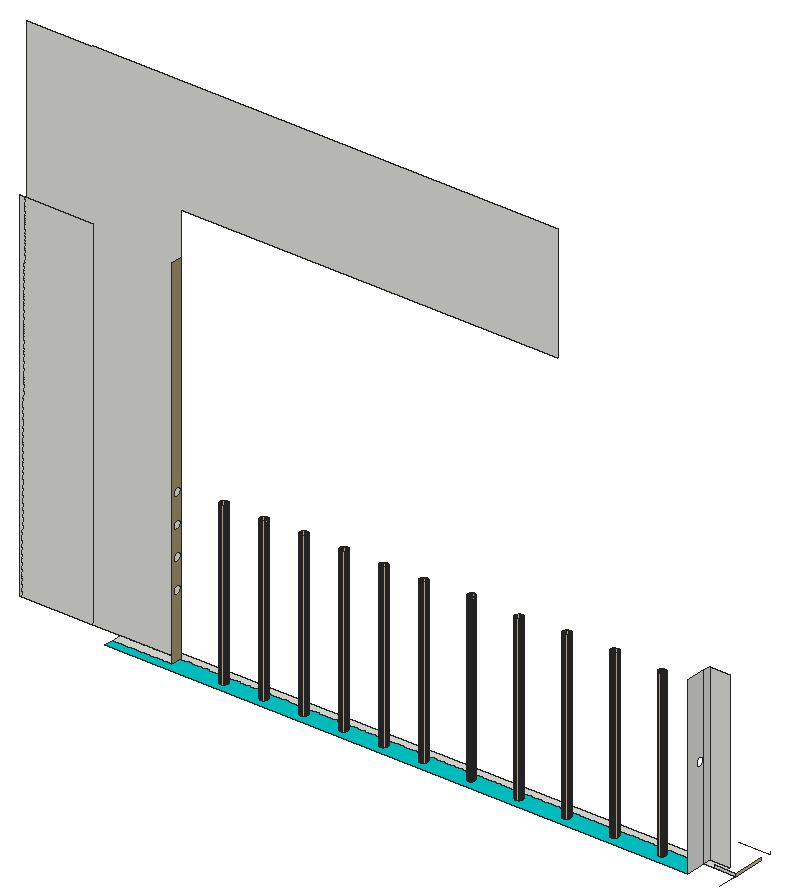
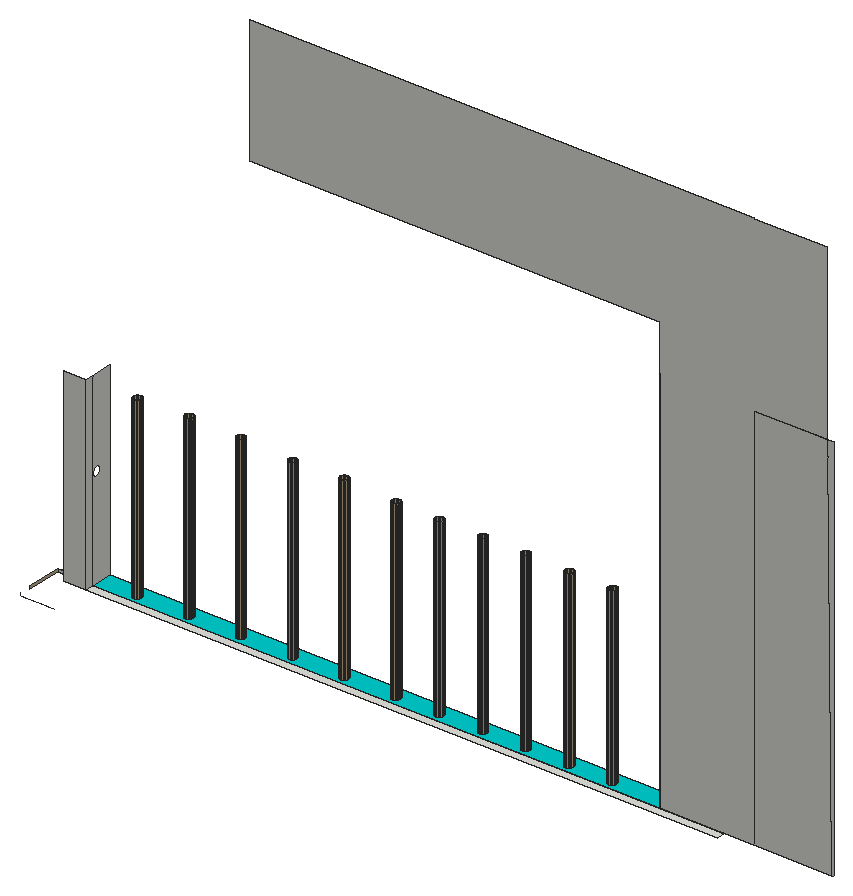
# SketchUp Ruby script. Lengths in inches.
U = 1.inch
M = Sketchup.active_model
def pt(a) = Geom::Point3d.new(a.map { |v| v * U })
def face(e, loops, mat)
  f = e.add_face(loops[0].map { |a| pt(a) })
  loops[1..].each { |l| e.add_face(l.map { |a| pt(a) }).erase! }
  f.material = f.back_material = mat if mat
  f
end
# faces: each face lists its corners as indices into pts; further lists are holes
def faces(e, pts, list, mat = nil) = list.each { |f| face(e, (f[0].is_a?(Array) ? f : [f]).map { |l| l.map { |i| pts[i] } }, mat) }
# xy, xz, yz: faces in a plane at the given z, y or x. An outline is a flat list of corners, or four numbers for a rectangle; further outlines are holes
def ring(l) = l.size == 4 ? [[l[0], l[1]], [l[2], l[1]], [l[2], l[3]], [l[0], l[3]]] : l.each_slice(2).to_a
def flat(e, list, mat, &to3) = list.each { |f| face(e, (f[0].is_a?(Array) ? f : [f]).map { |l| ring(l).map { |u, v| to3.(u, v) } }, mat) }
def xy(e, z, list, mat = nil) = flat(e, list, mat) { |x, y| [x, y, z] }
def xz(e, y, list, mat = nil) = flat(e, list, mat) { |x, z| [x, y, z] }
def yz(e, x, list, mat = nil) = flat(e, list, mat) { |y, z| [x, y, z] }
def lines(e, pts, list) = list.each { |a, b| e.add_line(pt(pts[a]), pt(pts[b])) }
# prism: a flat outline (further loops are holes) pulled along v
def prism(e, loops, v, mat = nil)
  f = face(e, loops, mat); d = Geom::Vector3d.new(v.map { |x| x * U })
  f.pushpull(f.normal.samedirection?(d) ? d.length : -d.length)
end
def box(e, o, s, mat = nil) = prism(e, [[o, [o[0] + s[0], o[1], o[2]], [o[0] + s[0], o[1] + s[1], o[2]], [o[0], o[1] + s[1], o[2]]]], [0, 0, s[2]], mat)
def at(x, y, z, deg = 0) = Geom::Transformation.translation(pt([x, y, z])) * Geom::Transformation.rotation(ORIGIN, Z_AXIS, deg.degrees)
def axes(o, x, y, z) = Geom::Transformation.new([*x, 0, *y, 0, *z, 0, *pt(o).to_a, 1])
def part(name) = M.definitions.add(name)
# library, detail: a bought-in or finely detailed component or shape, given as its bounding box
def library(name, o, s) = part(name).tap { |d| box(d.entities, o, s) }
def detail(e, o, s) = box(e.add_group.entities, o, s)
def put(e, d, t, mat = nil) = e.add_instance(d, t).tap { |i| i.material = mat if mat }
def group(e, t, mat = nil) = e.add_group.tap { |g| g.transformation = t; g.material = mat if mat }.entities
root = M.entities
M.materials.add("[Color H06]").color = [0, 204, 204]
M.materials.add("[Formica Beige]").color = [211, 187, 149]
M.materials.add("[Quartz Light Brown]").color = [199, 184, 152]
M.materials.add("[Wood Lumber ButtJoined]").color = [164, 152, 112]
xy(root,139.375,[[302.87,81.02,302.59,81.06,302.34,81.16,302.12,81.33,301.95,81.55,301.84,81.81,301.81,82.08,301.84,82.36,301.95,82.61,302.12,82.83,302.34,83,302.59,83.11,302.87,83.15,303.14,83.11,303.4,83,303.62,82.83,303.79,82.61,303.89,82.36,303.93,82.08,303.89,81.81,303.79,81.55,303.62,81.33,303.4,81.16,303.14,81.06],[314.06,81.02,313.78,81.06,313.52,81.16,313.3,81.33,313.13,81.55,313.03,81.81,312.99,82.08,313.03,82.36,313.13,82.61,313.3,82.83,313.52,83,313.78,83.11,314.06,83.15,314.33,83.11,314.59,83,314.81,82.83,314.98,82.61,315.08,82.36,315.12,82.08,315.08,81.81,314.98,81.55,314.81,81.33,314.59,81.16,314.33,81.06],[272.14,81.38,288.89,84.38],[272.14,84.38,435.38,86.51],[435.38,84.38,441.2,86.51]])
xy(root,139.375,[[[272.14,78.76,435.38,78.76,435.38,84.38,288.89,84.38,288.89,81.38,272.14,81.38],[314.06,81.02,313.78,81.06,313.52,81.16,313.3,81.33,313.13,81.55,313.03,81.81,312.99,82.08,313.03,82.36,313.13,82.61,313.3,82.83,313.52,83,313.78,83.11,314.06,83.15,314.33,83.11,314.59,83,314.81,82.83,314.98,82.61,315.08,82.36,315.12,82.08,315.08,81.81,314.98,81.55,314.81,81.33,314.59,81.16,314.33,81.06],[325.24,81.02,324.97,81.06,324.71,81.16,324.49,81.33,324.32,81.55,324.22,81.81,324.18,82.08,324.22,82.36,324.32,82.61,324.49,82.83,324.71,83,324.97,83.11,325.24,83.15,325.52,83.11,325.77,83,325.99,82.83,326.16,82.61,326.27,82.36,326.31,82.08,326.27,81.81,326.16,81.55,325.99,81.33,325.77,81.16,325.52,81.06],[336.43,81.02,336.16,81.06,335.9,81.16,335.68,81.33,335.51,81.55,335.4,81.81,335.37,82.08,335.4,82.36,335.51,82.61,335.68,82.83,335.9,83,336.16,83.11,336.43,83.15,336.71,83.11,336.96,83,337.18,82.83,337.35,82.61,337.46,82.36,337.49,82.08,337.46,81.81,337.35,81.55,337.18,81.33,336.96,81.16,336.71,81.06],[347.62,81.02,347.34,81.06,347.09,81.16,346.87,81.33,346.7,81.55,346.59,81.81,346.56,82.08,346.59,82.36,346.7,82.61,346.87,82.83,347.09,83,347.34,83.11,347.62,83.15,347.89,83.11,348.15,83,348.37,82.83,348.54,82.61,348.64,82.36,348.68,82.08,348.64,81.81,348.54,81.55,348.37,81.33,348.15,81.16,347.89,81.06],[358.81,81.02,358.53,81.06,358.27,81.16,358.05,81.33,357.88,81.55,357.78,81.81,357.74,82.08,357.78,82.36,357.88,82.61,358.05,82.83,358.27,83,358.53,83.11,358.81,83.15,359.08,83.11,359.34,83,359.56,82.83,359.73,82.61,359.83,82.36,359.87,82.08,359.83,81.81,359.73,81.55,359.56,81.33,359.34,81.16,359.08,81.06],[302.87,81.02,302.59,81.06,302.34,81.16,302.12,81.33,301.95,81.55,301.84,81.81,301.81,82.08,301.84,82.36,301.95,82.61,302.12,82.83,302.34,83,302.59,83.11,302.87,83.15,303.14,83.11,303.4,83,303.62,82.83,303.79,82.61,303.89,82.36,303.93,82.08,303.89,81.81,303.79,81.55,303.62,81.33,303.4,81.16,303.14,81.06],[372.18,81.02,371.91,81.06,371.65,81.16,371.43,81.33,371.26,81.55,371.15,81.81,371.12,82.08,371.15,82.36,371.26,82.61,371.43,82.83,371.65,83,371.91,83.11,372.18,83.15,372.46,83.11,372.71,83,372.93,82.83,373.1,82.61,373.21,82.36,373.24,82.08,373.21,81.81,373.1,81.55,372.93,81.33,372.71,81.16,372.46,81.06],[385.56,81.02,385.28,81.06,385.02,81.16,384.8,81.33,384.63,81.55,384.53,81.81,384.49,82.08,384.53,82.36,384.63,82.61,384.8,82.83,385.02,83,385.28,83.11,385.56,83.15,385.83,83.11,386.09,83,386.31,82.83,386.48,82.61,386.58,82.36,386.62,82.08,386.58,81.81,386.48,81.55,386.31,81.33,386.09,81.16,385.83,81.06],[398.93,81.02,398.66,81.06,398.4,81.16,398.18,81.33,398.01,81.55,397.9,81.81,397.87,82.08,397.9,82.36,398.01,82.61,398.18,82.83,398.4,83,398.66,83.11,398.93,83.15,399.21,83.11,399.46,83,399.68,82.83,399.85,82.61,399.96,82.36,399.99,82.08,399.96,81.81,399.85,81.55,399.68,81.33,399.46,81.16,399.21,81.06],[412.31,81.02,412.03,81.06,411.77,81.16,411.55,81.33,411.38,81.55,411.28,81.81,411.24,82.08,411.28,82.36,411.38,82.61,411.55,82.83,411.77,83,412.03,83.11,412.31,83.15,412.58,83.11,412.84,83,413.06,82.83,413.23,82.61,413.33,82.36,413.37,82.08,413.33,81.81,413.23,81.55,413.06,81.33,412.84,81.16,412.58,81.06],[425.68,81.02,425.41,81.06,425.15,81.16,424.93,81.33,424.76,81.55,424.65,81.81,424.62,82.08,424.65,82.36,424.76,82.61,424.93,82.83,425.15,83,425.41,83.11,425.68,83.15,425.96,83.11,426.21,83,426.43,82.83,426.6,82.61,426.71,82.36,426.74,82.08,426.71,81.81,426.6,81.55,426.43,81.33,426.21,81.16,425.96,81.06]]],"[Color H06]")
xz(root,84.38,[[243.82,139.375,243.82,240,245.26,240,244.42,139.375],[244.42,139.375,264.38,139.375,264.38,240,245.26,240],[264.38,139.375,264.38,240,245.63,240,245.63,284.5,264.38,284.5,264.38,284.625,394.7,284.625,394.7,252,288.89,252,288.89,139.375],[438.6,139.375,444.38,140.125]])
xz(root,86.51,[[435.38,139.375,441.2,188]])
yz(root,288.89,[[[81.38,139.375,84.38,240],[83.14,172.45,82.83,172.49,82.54,172.61,82.3,172.8,82.11,173.04,81.99,173.33,81.95,173.64,81.99,173.95,82.11,174.23,82.3,174.48,82.54,174.67,82.83,174.78,83.14,174.83,83.44,174.78,83.73,174.67,83.98,174.48,84.17,174.23,84.28,173.95,84.33,173.64,84.28,173.33,84.17,173.04,83.98,172.8,83.73,172.61,83.44,172.49],[83.14,164.26,82.83,164.3,82.54,164.42,82.3,164.61,82.11,164.86,81.99,165.14,81.95,165.45,81.99,165.76,82.11,166.04,82.3,166.29,82.54,166.48,82.83,166.6,83.14,166.64,83.44,166.6,83.73,166.48,83.98,166.29,84.17,166.04,84.28,165.76,84.33,165.45,84.28,165.14,84.17,164.86,83.98,164.61,83.73,164.42,83.44,164.3],[83.14,156.08,82.83,156.12,82.54,156.23,82.3,156.42,82.11,156.67,81.99,156.96,81.95,157.26,81.99,157.57,82.11,157.86,82.3,158.1,82.54,158.29,82.83,158.41,83.14,158.45,83.44,158.41,83.73,158.29,83.98,158.1,84.17,157.86,84.28,157.57,84.33,157.26,84.28,156.96,84.17,156.67,83.98,156.42,83.73,156.23,83.44,156.12],[83.14,180.64,82.83,180.68,82.54,180.8,82.3,180.99,82.11,181.23,81.99,181.52,81.95,181.83,81.99,182.13,82.11,182.42,82.3,182.67,82.54,182.85,82.83,182.97,83.14,183.01,83.44,182.97,83.73,182.85,83.98,182.67,84.17,182.42,84.28,182.13,84.33,181.83,84.28,181.52,84.17,181.23,83.98,180.99,83.73,180.8,83.44,180.68]]],"[Wood Lumber ButtJoined]")
yz(root,435.38,[[[78.76,139.375,84.38,188],[83.14,164.26,83.44,164.3,83.73,164.42,83.98,164.61,84.17,164.86,84.28,165.14,84.33,165.45,84.28,165.76,84.17,166.04,83.98,166.29,83.73,166.48,83.44,166.6,83.14,166.64,82.83,166.6,82.54,166.48,82.3,166.29,82.11,166.04,81.99,165.76,81.95,165.45,81.99,165.14,82.11,164.86,82.3,164.61,82.54,164.42,82.83,164.3]],[84.38,139.375,86.51,188]])
yz(root,444.38,[[84.38,139.375,93.38,140.125]],"[Quartz Light Brown]")
p = [[302.59,81.06,139.375],[302.87,81.02,139.375],[302.87,81.02,184.375],[302.59,81.06,184.375],[303.14,81.06,139.375],[303.14,81.06,184.375],
  [313.78,81.06,139.375],[314.06,81.02,139.375],[314.06,81.02,184.375],[313.78,81.06,184.375],[314.33,81.06,139.375],[314.33,81.06,184.375],
  [324.97,81.06,139.375],[325.24,81.02,139.375],[325.24,81.02,184.625],[324.97,81.06,184.625],[325.52,81.06,139.375],[325.52,81.06,184.625],
  [336.16,81.06,139.375],[336.43,81.02,139.375],[336.43,81.02,184.625],[336.16,81.06,184.625],[336.71,81.06,139.375],[336.71,81.06,184.625],
  [347.34,81.06,139.375],[347.62,81.02,139.375],[347.62,81.02,184.625],[347.34,81.06,184.625],[347.89,81.06,139.375],[347.89,81.06,184.625],
  [358.53,81.06,139.375],[358.81,81.02,139.375],[358.81,81.02,184.75],[358.53,81.06,184.75],[359.08,81.06,139.375],[359.08,81.06,184.75],
  [371.91,81.06,139.375],[372.18,81.02,139.375],[372.18,81.02,185.5625],[371.91,81.06,185.5625],[372.46,81.06,139.375],[372.46,81.06,185.5625],
  [385.28,81.06,139.375],[385.56,81.02,139.375],[385.56,81.02,184.9375],[385.28,81.06,184.9375],[385.83,81.06,139.375],[385.83,81.06,184.9375],
  [398.66,81.06,139.375],[398.93,81.02,139.375],[398.93,81.02,185.625],[398.66,81.06,185.625],[399.21,81.06,139.375],[399.21,81.06,185.625],
  [412.03,81.06,139.375],[412.31,81.02,139.375],[412.31,81.02,185.8125],[412.03,81.06,185.8125],[412.58,81.06,139.375],[412.58,81.06,185.8125],
  [425.41,81.06,139.375],[425.68,81.02,139.375],[425.68,81.02,185.3125],[425.41,81.06,185.3125],[425.96,81.06,139.375],[425.96,81.06,185.3125],
  [302.34,81.16,139.375],[302.34,81.16,184.375],[303.4,81.16,139.375],[303.4,81.16,184.375],[313.52,81.16,139.375],[313.52,81.16,184.375],
  [314.59,81.16,139.375],[314.59,81.16,184.375],[324.71,81.16,139.375],[324.71,81.16,184.625],[325.77,81.16,139.375],[325.77,81.16,184.625],
  [335.9,81.16,139.375],[335.9,81.16,184.625],[336.96,81.16,139.375],[336.96,81.16,184.625],[347.09,81.16,139.375],[347.09,81.16,184.625],
  [348.15,81.16,139.375],[348.15,81.16,184.625],[358.27,81.16,139.375],[358.27,81.16,184.75],[359.34,81.16,139.375],[359.34,81.16,184.75],
  [371.65,81.16,139.375],[371.65,81.16,185.5625],[372.71,81.16,139.375],[372.71,81.16,185.5625],[385.02,81.16,139.375],[385.02,81.16,184.9375],
  [386.09,81.16,139.375],[386.09,81.16,184.9375],[398.4,81.16,139.375],[398.4,81.16,185.625],[399.46,81.16,139.375],[399.46,81.16,185.625],
  [411.77,81.16,139.375],[411.77,81.16,185.8125],[412.84,81.16,139.375],[412.84,81.16,185.8125],[425.15,81.16,139.375],[425.15,81.16,185.3125],
  [426.21,81.16,139.375],[426.21,81.16,185.3125],[302.12,81.33,139.375],[302.12,81.33,184.375],[303.62,81.33,139.375],[303.62,81.33,184.375],
  [313.3,81.33,139.375],[313.3,81.33,184.375],[314.81,81.33,139.375],[314.81,81.33,184.375],[324.49,81.33,139.375],[324.49,81.33,184.625],
  [325.99,81.33,139.375],[325.99,81.33,184.625],[335.68,81.33,139.375],[335.68,81.33,184.625],[337.18,81.33,139.375],[337.18,81.33,184.625],
  [346.87,81.33,139.375],[346.87,81.33,184.625],[348.37,81.33,139.375],[348.37,81.33,184.625],[358.05,81.33,139.375],[358.05,81.33,184.75],
  [359.56,81.33,139.375],[359.56,81.33,184.75],[371.43,81.33,139.375],[371.43,81.33,185.5625],[372.93,81.33,139.375],[372.93,81.33,185.5625],
  [384.8,81.33,139.375],[384.8,81.33,184.9375],[386.31,81.33,139.375],[386.31,81.33,184.9375],[398.18,81.33,139.375],[398.18,81.33,185.625],
  [399.68,81.33,139.375],[399.68,81.33,185.625],[411.55,81.33,139.375],[411.55,81.33,185.8125],[413.06,81.33,139.375],[413.06,81.33,185.8125],
  [424.93,81.33,139.375],[424.93,81.33,185.3125],[426.43,81.33,139.375],[426.43,81.33,185.3125],[301.95,81.55,139.375],[301.95,81.55,184.375],
  [303.79,81.55,139.375],[303.79,81.55,184.375],[313.13,81.55,139.375],[313.13,81.55,184.375],[314.98,81.55,139.375],[314.98,81.55,184.375],
  [324.32,81.55,139.375],[324.32,81.55,184.625],[326.16,81.55,139.375],[326.16,81.55,184.625],[335.51,81.55,139.375],[335.51,81.55,184.625],
  [337.35,81.55,139.375],[337.35,81.55,184.625],[346.7,81.55,139.375],[346.7,81.55,184.625],[348.54,81.55,139.375],[348.54,81.55,184.625],
  [357.88,81.55,139.375],[357.88,81.55,184.75],[359.73,81.55,139.375],[359.73,81.55,184.75],[371.26,81.55,139.375],[371.26,81.55,185.5625],
  [373.1,81.55,139.375],[373.1,81.55,185.5625],[384.63,81.55,139.375],[384.63,81.55,184.9375],[386.48,81.55,139.375],[386.48,81.55,184.9375],
  [398.01,81.55,139.375],[398.01,81.55,185.625],[399.85,81.55,139.375],[399.85,81.55,185.625],[411.38,81.55,139.375],[411.38,81.55,185.8125],
  [413.23,81.55,139.375],[413.23,81.55,185.8125],[424.76,81.55,139.375],[424.76,81.55,185.3125],[426.6,81.55,139.375],[426.6,81.55,185.3125],
  [301.84,81.81,139.375],[301.84,81.81,184.375],[303.89,81.81,139.375],[303.89,81.81,184.375],[313.03,81.81,139.375],[313.03,81.81,184.375],
  [315.08,81.81,139.375],[315.08,81.81,184.375],[324.22,81.81,139.375],[324.22,81.81,184.625],[326.27,81.81,139.375],[326.27,81.81,184.625],
  [335.4,81.81,139.375],[335.4,81.81,184.625],[337.46,81.81,139.375],[337.46,81.81,184.625],[346.59,81.81,139.375],[346.59,81.81,184.625],
  [348.64,81.81,139.375],[348.64,81.81,184.625],[357.78,81.81,139.375],[357.78,81.81,184.75],[359.83,81.81,139.375],[359.83,81.81,184.75],
  [371.15,81.81,139.375],[371.15,81.81,185.5625],[373.21,81.81,139.375],[373.21,81.81,185.5625],[384.53,81.81,139.375],[384.53,81.81,184.9375],
  [386.58,81.81,139.375],[386.58,81.81,184.9375],[397.9,81.81,139.375],[397.9,81.81,185.625],[399.96,81.81,139.375],[399.96,81.81,185.625],
  [411.28,81.81,139.375],[411.28,81.81,185.8125],[413.33,81.81,139.375],[413.33,81.81,185.8125],[424.65,81.81,139.375],[424.65,81.81,185.3125],
  [426.71,81.81,139.375],[426.71,81.81,185.3125],[301.81,82.08,139.375],[301.81,82.08,184.375],[303.93,82.08,139.375],[303.93,82.08,184.375],
  [312.99,82.08,139.375],[312.99,82.08,184.375],[315.12,82.08,139.375],[315.12,82.08,184.375],[324.18,82.08,139.375],[324.18,82.08,184.625],
  [326.31,82.08,139.375],[326.31,82.08,184.625],[335.37,82.08,139.375],[335.37,82.08,184.625],[337.49,82.08,139.375],[337.49,82.08,184.625],
  [346.56,82.08,139.375],[346.56,82.08,184.625],[348.68,82.08,139.375],[348.68,82.08,184.625],[357.74,82.08,139.375],[357.74,82.08,184.75],
  [359.87,82.08,139.375],[359.87,82.08,184.75],[371.12,82.08,139.375],[371.12,82.08,185.5625],[373.24,82.08,139.375],[373.24,82.08,185.5625],
  [384.49,82.08,139.375],[384.49,82.08,184.9375],[386.62,82.08,139.375],[386.62,82.08,184.9375],[397.87,82.08,139.375],[397.87,82.08,185.625],
  [399.99,82.08,139.375],[399.99,82.08,185.625],[411.24,82.08,139.375],[411.24,82.08,185.8125],[413.37,82.08,139.375],[413.37,82.08,185.8125],
  [424.62,82.08,139.375],[424.62,82.08,185.3125],[426.74,82.08,139.375],[426.74,82.08,185.3125],[301.84,82.36,139.375],[301.84,82.36,184.375],
  [303.89,82.36,139.375],[303.89,82.36,184.375],[313.03,82.36,139.375],[313.03,82.36,184.375],[315.08,82.36,139.375],[315.08,82.36,184.375],
  [324.22,82.36,139.375],[324.22,82.36,184.625],[326.27,82.36,139.375],[326.27,82.36,184.625],[335.4,82.36,139.375],[335.4,82.36,184.625],
  [337.46,82.36,139.375],[337.46,82.36,184.625],[346.59,82.36,139.375],[346.59,82.36,184.625],[348.64,82.36,139.375],[348.64,82.36,184.625],
  [357.78,82.36,139.375],[357.78,82.36,184.75],[359.83,82.36,139.375],[359.83,82.36,184.75],[371.15,82.36,139.375],[371.15,82.36,185.5625],
  [373.21,82.36,139.375],[373.21,82.36,185.5625],[384.53,82.36,139.375],[384.53,82.36,184.9375],[386.58,82.36,139.375],[386.58,82.36,184.9375],
  [397.9,82.36,139.375],[397.9,82.36,185.625],[399.96,82.36,139.375],[399.96,82.36,185.625],[411.28,82.36,139.375],[411.28,82.36,185.8125],
  [413.33,82.36,139.375],[413.33,82.36,185.8125],[424.65,82.36,139.375],[424.65,82.36,185.3125],[426.71,82.36,139.375],[426.71,82.36,185.3125],
  [301.95,82.61,139.375],[301.95,82.61,184.375],[303.79,82.61,139.375],[303.79,82.61,184.375],[313.13,82.61,139.375],[313.13,82.61,184.375],
  [314.98,82.61,139.375],[314.98,82.61,184.375],[324.32,82.61,139.375],[324.32,82.61,184.625],[326.16,82.61,139.375],[326.16,82.61,184.625],
  [335.51,82.61,139.375],[335.51,82.61,184.625],[337.35,82.61,139.375],[337.35,82.61,184.625],[346.7,82.61,139.375],[346.7,82.61,184.625],
  [348.54,82.61,139.375],[348.54,82.61,184.625],[357.88,82.61,139.375],[357.88,82.61,184.75],[359.73,82.61,139.375],[359.73,82.61,184.75],
  [371.26,82.61,139.375],[371.26,82.61,185.5625],[373.1,82.61,139.375],[373.1,82.61,185.5625],[384.63,82.61,139.375],[384.63,82.61,184.9375],
  [386.48,82.61,139.375],[386.48,82.61,184.9375],[398.01,82.61,139.375],[398.01,82.61,185.625],[399.85,82.61,139.375],[399.85,82.61,185.625],
  [411.38,82.61,139.375],[411.38,82.61,185.8125],[413.23,82.61,139.375],[413.23,82.61,185.8125],[424.76,82.61,139.375],[424.76,82.61,185.3125],
  [426.6,82.61,139.375],[426.6,82.61,185.3125],[302.12,82.83,139.375],[302.12,82.83,184.375],[303.62,82.83,139.375],[303.62,82.83,184.375],
  [313.3,82.83,139.375],[313.3,82.83,184.375],[314.81,82.83,139.375],[314.81,82.83,184.375],[324.49,82.83,139.375],[324.49,82.83,184.625],
  [325.99,82.83,139.375],[325.99,82.83,184.625],[335.68,82.83,139.375],[335.68,82.83,184.625],[337.18,82.83,139.375],[337.18,82.83,184.625],
  [346.87,82.83,139.375],[346.87,82.83,184.625],[348.37,82.83,139.375],[348.37,82.83,184.625],[358.05,82.83,139.375],[358.05,82.83,184.75],
  [359.56,82.83,139.375],[359.56,82.83,184.75],[371.43,82.83,139.375],[371.43,82.83,185.5625],[372.93,82.83,139.375],[372.93,82.83,185.5625],
  [384.8,82.83,139.375],[384.8,82.83,184.9375],[386.31,82.83,139.375],[386.31,82.83,184.9375],[398.18,82.83,139.375],[398.18,82.83,185.625],
  [399.68,82.83,139.375],[399.68,82.83,185.625],[411.55,82.83,139.375],[411.55,82.83,185.8125],[413.06,82.83,139.375],[413.06,82.83,185.8125],
  [424.93,82.83,139.375],[424.93,82.83,185.3125],[426.43,82.83,139.375],[426.43,82.83,185.3125],[302.34,83,139.375],[302.34,83,184.375],
  [303.4,83,139.375],[303.4,83,184.375],[313.52,83,139.375],[313.52,83,184.375],[314.59,83,139.375],[314.59,83,184.375],
  [324.71,83,139.375],[324.71,83,184.625],[325.77,83,139.375],[325.77,83,184.625],[335.9,83,139.375],[335.9,83,184.625],
  [336.96,83,139.375],[336.96,83,184.625],[347.09,83,139.375],[347.09,83,184.625],[348.15,83,139.375],[348.15,83,184.625],
  [358.27,83,139.375],[358.27,83,184.75],[359.34,83,139.375],[359.34,83,184.75],[371.65,83,139.375],[371.65,83,185.5625],
  [372.71,83,139.375],[372.71,83,185.5625],[385.02,83,139.375],[385.02,83,184.9375],[386.09,83,139.375],[386.09,83,184.9375],
  [398.4,83,139.375],[398.4,83,185.625],[399.46,83,139.375],[399.46,83,185.625],[411.77,83,139.375],[411.77,83,185.8125],
  [412.84,83,139.375],[412.84,83,185.8125],[425.15,83,139.375],[425.15,83,185.3125],[426.21,83,139.375],[426.21,83,185.3125],
  [302.59,83.11,139.375],[302.59,83.11,184.375],[303.14,83.11,139.375],[303.14,83.11,184.375],[313.78,83.11,139.375],[313.78,83.11,184.375],
  [314.33,83.11,139.375],[314.33,83.11,184.375],[324.97,83.11,139.375],[324.97,83.11,184.625],[325.52,83.11,139.375],[325.52,83.11,184.625],
  [336.16,83.11,139.375],[336.16,83.11,184.625],[336.71,83.11,139.375],[336.71,83.11,184.625],[347.34,83.11,139.375],[347.34,83.11,184.625],
  [347.89,83.11,139.375],[347.89,83.11,184.625],[358.53,83.11,139.375],[358.53,83.11,184.75],[359.08,83.11,139.375],[359.08,83.11,184.75],
  [371.91,83.11,139.375],[371.91,83.11,185.5625],[372.46,83.11,139.375],[372.46,83.11,185.5625],[385.28,83.11,139.375],[385.28,83.11,184.9375],
  [385.83,83.11,139.375],[385.83,83.11,184.9375],[398.66,83.11,139.375],[398.66,83.11,185.625],[399.21,83.11,139.375],[399.21,83.11,185.625],
  [412.03,83.11,139.375],[412.03,83.11,185.8125],[412.58,83.11,139.375],[412.58,83.11,185.8125],[425.41,83.11,139.375],[425.41,83.11,185.3125],
  [425.96,83.11,139.375],[425.96,83.11,185.3125],[302.87,83.15,139.375],[302.87,83.15,184.375],[314.06,83.15,139.375],[314.06,83.15,184.375],
  [325.24,83.15,139.375],[325.24,83.15,184.625],[336.43,83.15,139.375],[336.43,83.15,184.625],[347.62,83.15,139.375],[347.62,83.15,184.625],
  [358.81,83.15,139.375],[358.81,83.15,184.75],[372.18,83.15,139.375],[372.18,83.15,185.5625],[385.56,83.15,139.375],[385.56,83.15,184.9375],
  [398.93,83.15,139.375],[398.93,83.15,185.625],[412.31,83.15,139.375],[412.31,83.15,185.8125],[425.68,83.15,139.375],[425.68,83.15,185.3125],
  [444.38,96.7,139.375],[444.38,96.7,140.125],[435.38,96.7,139.375],[444.38,78.76,139.375],[444.38,84.38,139.375]]
faces(root,p,[[0,1,2,3],[1,4,5,2],[6,7,8,9],[7,10,11,8],[12,13,14,15],[13,16,17,14],[18,19,20,21],[19,22,23,20],
  [24,25,26,27],[25,28,29,26],[30,31,32,33],[31,34,35,32],[36,37,38,39],[37,40,41,38],[42,43,44,45],[43,46,47,44],
  [48,49,50,51],[49,52,53,50],[54,55,56,57],[55,58,59,56],[60,61,62,63],[61,64,65,62],[66,0,3,67],[4,68,69,5],
  [70,6,9,71],[10,72,73,11],[74,12,15,75],[16,76,77,17],[78,18,21,79],[22,80,81,23],[82,24,27,83],[28,84,85,29],
  [86,30,33,87],[34,88,89,35],[90,36,39,91],[40,92,93,41],[94,42,45,95],[46,96,97,47],[98,48,51,99],[52,100,101,53],
  [102,54,57,103],[58,104,105,59],[106,60,63,107],[64,108,109,65],[110,66,67,111],[68,112,113,69],[114,70,71,115],[72,116,117,73],
  [118,74,75,119],[76,120,121,77],[122,78,79,123],[80,124,125,81],[126,82,83,127],[84,128,129,85],[130,86,87,131],[88,132,133,89],
  [134,90,91,135],[92,136,137,93],[138,94,95,139],[96,140,141,97],[142,98,99,143],[100,144,145,101],[146,102,103,147],[104,148,149,105],
  [150,106,107,151],[108,152,153,109],[154,110,111,155],[112,156,157,113],[158,114,115,159],[116,160,161,117],[162,118,119,163],[120,164,165,121],
  [166,122,123,167],[124,168,169,125],[170,126,127,171],[128,172,173,129],[174,130,131,175],[132,176,177,133],[178,134,135,179],[136,180,181,137],
  [182,138,139,183],[140,184,185,141],[186,142,143,187],[144,188,189,145],[190,146,147,191],[148,192,193,149],[194,150,151,195],[152,196,197,153],
  [198,154,155,199],[156,200,201,157],[202,158,159,203],[160,204,205,161],[206,162,163,207],[164,208,209,165],[210,166,167,211],[168,212,213,169],
  [214,170,171,215],[172,216,217,173],[218,174,175,219],[176,220,221,177],[222,178,179,223],[180,224,225,181],[226,182,183,227],[184,228,229,185],
  [230,186,187,231],[188,232,233,189],[234,190,191,235],[192,236,237,193],[238,194,195,239],[196,240,241,197],[242,198,199,243],[200,244,245,201],
  [246,202,203,247],[204,248,249,205],[250,206,207,251],[208,252,253,209],[254,210,211,255],[212,256,257,213],[258,214,215,259],[216,260,261,217],
  [262,218,219,263],[220,264,265,221],[266,222,223,267],[224,268,269,225],[270,226,227,271],[228,272,273,229],[274,230,231,275],[232,276,277,233],
  [278,234,235,279],[236,280,281,237],[282,238,239,283],[240,284,285,241],[286,242,243,287],[244,288,289,245],[290,246,247,291],[248,292,293,249],
  [294,250,251,295],[252,296,297,253],[298,254,255,299],[256,300,301,257],[302,258,259,303],[260,304,305,261],[306,262,263,307],[264,308,309,265],
  [310,266,267,311],[268,312,313,269],[314,270,271,315],[272,316,317,273],[318,274,275,319],[276,320,321,277],[322,278,279,323],[280,324,325,281],
  [326,282,283,327],[284,328,329,285],[330,286,287,331],[288,332,333,289],[334,290,291,335],[292,336,337,293],[338,294,295,339],[296,340,341,297],
  [342,298,299,343],[300,344,345,301],[346,302,303,347],[304,348,349,305],[350,306,307,351],[308,352,353,309],[354,310,311,355],[312,356,357,313],
  [358,314,315,359],[316,360,361,317],[362,318,319,363],[320,364,365,321],[366,322,323,367],[324,368,369,325],[370,326,327,371],[328,372,373,329],
  [374,330,331,375],[332,376,377,333],[378,334,335,379],[336,380,381,337],[382,338,339,383],[340,384,385,341],[386,342,343,387],[344,388,389,345],
  [390,346,347,391],[348,392,393,349],[394,350,351,395],[352,396,397,353],[398,354,355,399],[356,400,401,357],[402,358,359,403],[360,404,405,361],
  [406,362,363,407],[364,408,409,365],[410,366,367,411],[368,412,413,369],[414,370,371,415],[372,416,417,373],[418,374,375,419],[376,420,421,377],
  [422,378,379,423],[380,424,425,381],[426,382,383,427],[384,428,429,385],[430,386,387,431],[388,432,433,389],[434,390,391,435],[392,436,437,393],
  [438,394,395,439],[396,440,441,397],[442,398,399,443],[400,444,445,401],[446,402,403,447],[404,448,449,405],[450,406,407,451],[408,452,453,409],
  [454,410,411,455],[412,456,457,413],[458,414,415,459],[416,460,461,417],[462,418,419,463],[420,464,465,421],[466,422,423,467],[424,468,469,425],
  [470,426,427,471],[428,472,473,429],[474,430,431,475],[432,476,477,433],[478,434,435,479],[436,480,481,437],[482,438,439,483],[440,484,485,441],
  [486,442,443,487],[444,488,489,445],[490,446,447,491],[448,492,493,449],[494,450,451,495],[452,496,497,453],[498,454,455,499],[456,500,501,457],
  [502,458,459,503],[460,504,505,461],[506,462,463,507],[464,506,507,465],[508,466,467,509],[468,508,509,469],[510,470,471,511],[472,510,511,473],
  [512,474,475,513],[476,512,513,477],[514,478,479,515],[480,514,515,481],[516,482,483,517],[484,516,517,485],[518,486,487,519],[488,518,519,489],
  [520,490,491,521],[492,520,521,493],[522,494,495,523],[496,522,523,497],[524,498,499,525],[500,524,525,501],[526,502,503,527],[504,526,527,505]],"[Formica Beige]")
lines(root,p,[[528,529],[530,528],[531,532]])
